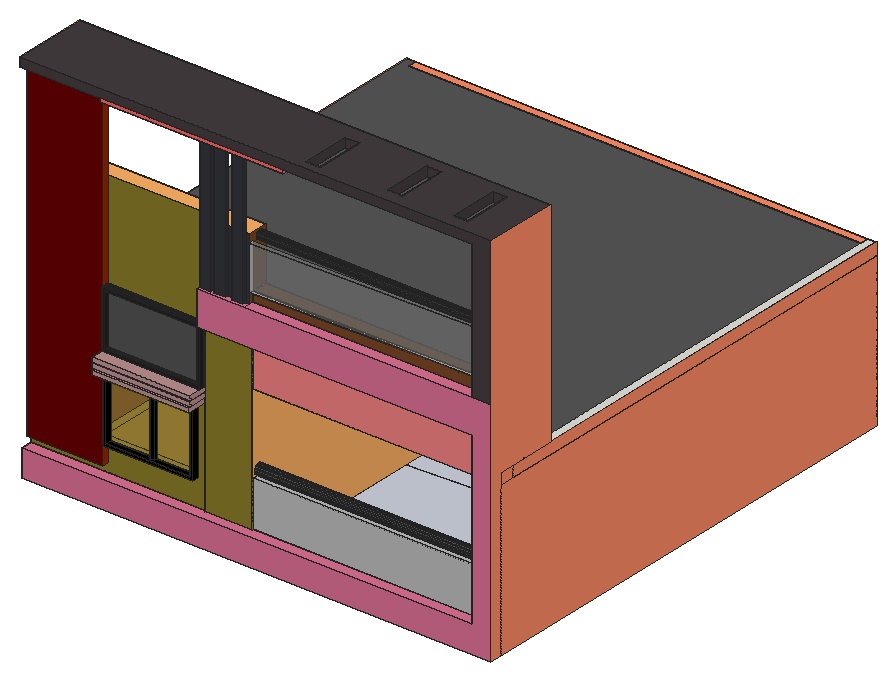
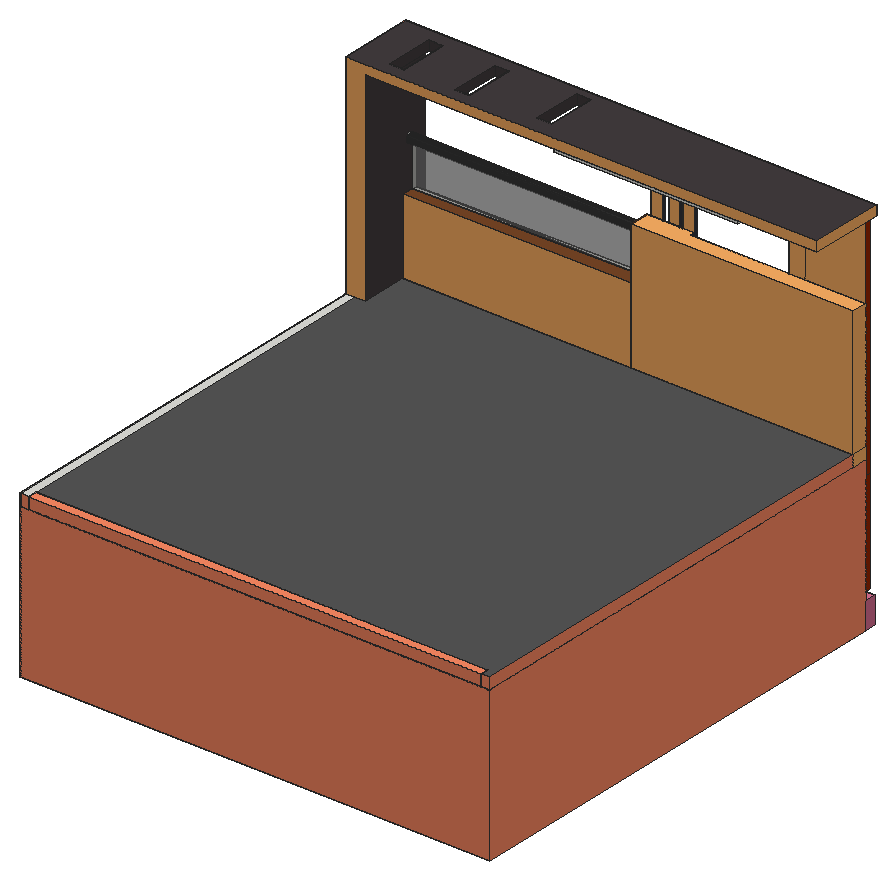
# SketchUp Ruby script. Lengths in inches.
U = 1.inch
M = Sketchup.active_model
def pt(a) = Geom::Point3d.new(a.map { |v| v * U })
def face(e, loops, mat)
  f = e.add_face(loops[0].map { |a| pt(a) })
  loops[1..].each { |l| e.add_face(l.map { |a| pt(a) }).erase! }
  f.material = f.back_material = mat if mat
  f
end
# faces: each face lists its corners as indices into pts; further lists are holes
def faces(e, pts, list, mat = nil) = list.each { |f| face(e, (f[0].is_a?(Array) ? f : [f]).map { |l| l.map { |i| pts[i] } }, mat) }
# xy, xz, yz: faces in a plane at the given z, y or x. An outline is a flat list of corners, or four numbers for a rectangle; further outlines are holes
def ring(l) = l.size == 4 ? [[l[0], l[1]], [l[2], l[1]], [l[2], l[3]], [l[0], l[3]]] : l.each_slice(2).to_a
def flat(e, list, mat, &to3) = list.each { |f| face(e, (f[0].is_a?(Array) ? f : [f]).map { |l| ring(l).map { |u, v| to3.(u, v) } }, mat) }
def xy(e, z, list, mat = nil) = flat(e, list, mat) { |x, y| [x, y, z] }
def xz(e, y, list, mat = nil) = flat(e, list, mat) { |x, z| [x, y, z] }
def yz(e, x, list, mat = nil) = flat(e, list, mat) { |y, z| [x, y, z] }
def lines(e, pts, list) = list.each { |a, b| e.add_line(pt(pts[a]), pt(pts[b])) }
# prism: a flat outline (further loops are holes) pulled along v
def prism(e, loops, v, mat = nil)
  f = face(e, loops, mat); d = Geom::Vector3d.new(v.map { |x| x * U })
  f.pushpull(f.normal.samedirection?(d) ? d.length : -d.length)
end
def box(e, o, s, mat = nil) = prism(e, [[o, [o[0] + s[0], o[1], o[2]], [o[0] + s[0], o[1] + s[1], o[2]], [o[0], o[1] + s[1], o[2]]]], [0, 0, s[2]], mat)
def at(x, y, z, deg = 0) = Geom::Transformation.translation(pt([x, y, z])) * Geom::Transformation.rotation(ORIGIN, Z_AXIS, deg.degrees)
def axes(o, x, y, z) = Geom::Transformation.new([*x, 0, *y, 0, *z, 0, *pt(o).to_a, 1])
def part(name) = M.definitions.add(name)
# library, detail: a bought-in or finely detailed component or shape, given as its bounding box
def library(name, o, s) = part(name).tap { |d| box(d.entities, o, s) }
def detail(e, o, s) = box(e.add_group.entities, o, s)
def put(e, d, t, mat = nil) = e.add_instance(d, t).tap { |i| i.material = mat if mat }
def group(e, t, mat = nil) = e.add_group.tap { |g| g.transformation = t; g.material = mat if mat }.entities
root = M.entities
M.materials.add("[0001_PaleVioletRed]").color = [219, 112, 147]
M.materials.add("[0013_LightCoral]").color = [240, 128, 128]
M.materials.add("[0119_RosyBrown]").color = [188, 143, 143]
M.materials.add("[0135_DarkGray]").color = [81, 81, 81]
M.materials.add("[0136_Charcoal]").color = [35, 35, 35]
M.materials.add("[Asphalt New]").color = [67, 60, 62]
M.materials.add("[Color A03]").color = [255, 101, 101]
M.materials.add("[Color A08]").color = [102, 0, 0]
M.materials.add("[Color B03]").color = [255, 140, 101]
M.materials.add("[Color B07]").color = [153, 38, 0]
M.materials.add("[Color C03]").color = [255, 178, 101]
M.materials.add("[Color M06]").color = [86, 86, 86]
M.materials.add("[Color M07]").color = [58, 58, 58]
M.materials.add("[Color M09]").color = [0, 0, 0]
M.materials.add("[Formica Laminate Dark]").color = [50, 53, 60]
M.materials.add("[Marble Carrara Floor Tile]").color = [204, 208, 219]
M.materials.add("[Mirror 01]").color = [185, 185, 185]
M.materials.add("[Translucent Glass Dark Green]").color = [62, 91, 5]
M.materials["[Translucent Glass Dark Green]"].alpha = 0.5
M.materials.add("[Translucent Glass Gray]").color = [128, 128, 128]
M.materials["[Translucent Glass Gray]"].alpha = 0.5
M.materials.add("[Wood Floor]").color = [155, 105, 61]
M.materials.add("[Wood Plywood Knots]").color = [137, 122, 41]
M.materials.add("[Wood Veneer 01]").color = [120, 70, 37]
c1 = library("glass+door",[0,-2.95,0],[39.37,5.9,82.68])
xy(root,156,[[472.5,7.75,481.5,19.75],[228.3125,215.25,228.3125,331.6875,272.65,331.6875,272.65,337.6875,222.3125,337.6875,222.3125,331.34],[430.11,331.6875,467.13,331.6875,466.82,337.6875,430.11,337.6875]])
xy(root,156,[[1.5,7.75,10.5,19.75],[10.5,7.75,10.5,19.75,179.9375,19.75,179.9375,18.75,228.3125,18.75,228.3125,19.75,472.5,19.75,472.5,7.75]],"[0001_PaleVioletRed]")
xy(root,156,[[[1.5,19.75,481.5,499.75],[10.5,28.75,472.5,28.75,472.5,331.6875,467.13,331.6875,466.82,337.6875,472.5,337.6875,472.5,490.75,10.5,490.75,10.5,221.25,222.3125,221.25,222.3125,331.34,228.3125,215.25,10.5,215.25]],[10.5,28.75,228.3125,215.25],[228.3125,28.75,228.3125,215.25,472.5,227.87,472.5,28.75]],"[Color C03]")
xy(root,156,[[228.3125,215.25,472.5,227.87,467.13,331.6875,430.11,331.6875,430.11,337.6875,472.5,337.6875,472.5,490.75,10.5,490.75,10.5,221.25,222.3125,221.25,222.3125,337.6875,272.65,337.6875,272.65,331.6875,228.3125,331.6875],[472.5,227.87,472.5,331.6875,467.13,331.6875]],"[Marble Carrara Floor Tile]")
xy(root,156.5,[[228.3125,28.75,472.5,28.75,472.5,227.87,228.3125,215.25]],"[Marble Carrara Floor Tile]")
xy(root,183.125,[[10.5,19.75,228.3125,28.75]])
xy(root,183.125,[[1.5,7.75,461.5625,19.75]],"[0001_PaleVioletRed]")
xy(root,191.625,[[1.5,13.75,63.75,19.75],[63.75,13.75,79.5,19.75]])
xy(root,210.02,[[79.5,13.75,171.875,19.75]])
xy(root,213.02,[[125.6875,16.75,129.85,19.75]])
xy(root,213.02,[[82.5,13.75,168.875,13.75,168.875,19.75,129.85,19.75,129.85,16.75,125.6875,16.75,125.6875,19.75,82.5,19.75]],"[Color M09]")
xy(root,230.125,[[228.3125,19.75,472.5,28.75]],"[Mirror 01]")
xy(root,253.3125,[[272.65,331.6875,430.11,337.6875]])
xy(root,271.2,[[125.6875,16.75,129.85,19.75]])
xy(root,271.2,[[82.5,13.75,82.5,19.75,125.6875,19.75,125.6875,16.75,129.85,16.75,129.85,19.75,168.875,19.75,168.875,13.75]],"[Color M09]")
xy(root,274.2,[[79.5,13.75,171.875,19.75]],"[Color M09]")
xy(root,281.13,[[79.5,0,178.52,19.75]],"[0119_RosyBrown]")
xy(root,285.75,[[79.5,0,178.45,19.75]],"[0119_RosyBrown]")
xy(root,286.88,[[79.5,0,180,19.75]],"[0119_RosyBrown]")
xy(root,291.5,[[79.5,0,179.9375,19.75]],"[0119_RosyBrown]")
xy(root,292.57,[[79.5,0,180,19.75]],"[0119_RosyBrown]")
xy(root,297.1875,[[79.5,12.4375,179.9375,15.4375],[79.5,15.4375,179.9375,19.75]])
xy(root,297.1875,[[79.5,0,179.9375,12.4375]],"[0119_RosyBrown]")
xy(root,300.53,[[82.84,12.4375,176.6,15.4375]],"[0136_Charcoal]")
xy(root,310.125,[[228.3125,35.87,472.5,331.6875]],"[0013_LightCoral]")
xy(root,311.9375,[[[1.5,35.87,1.5,499.75,481.5,499.75,481.5,35.87,472.5,35.87,472.5,331.6875,228.3125,331.6875,228.3125,35.87],[10.5,221.25,222.3125,221.25,222.3125,337.6875,472.5,337.6875,472.5,490.75,10.5,490.75]]])
xy(root,312,[[1.5,19.75,228.3125,35.87],[472.5,19.75,481.5,35.87],[1.5,35.87,228.3125,35.87,228.3125,221.25,10.5,221.25,10.5,490.75,10.375,490.75,10.375,499.75,1.5,499.75],[228.3125,35.87,472.5,221.25],[472.5,35.87,472.6875,221.25],
  [472.6875,35.87,481.25,499.75],[481.25,35.87,481.5,499.75],[10.5,221.25,10.5,490.75,472.5,490.75,472.5,337.6875,222.3125,337.6875,222.3125,221.25],[222.3125,221.25,228.3125,221.25,228.3125,331.6875,472.6875,331.6875,472.6875,337.6875,222.3125,337.6875],[228.3125,221.25,472.5,331.6875],
  [472.5,221.25,472.6875,331.6875],[472.5,337.6875,472.6875,490.75],[10.375,490.75,472.6875,499.75]])
xy(root,312,[[228.3125,19.75,472.5,35.87]],"[0013_LightCoral]")
xy(root,324,[[461.5625,19.75,481.5,35.87],[472.6875,35.87,481.25,83.5],[481.25,35.87,481.5,83.5],[472.6875,83.5,481.25,499.75],[481.25,83.5,481.5,499.75]])
xy(root,324,[[461.5625,35.87,472.6875,83.5],[10.375,490.75,472.6875,499.75]],"[Color B03]")
xy(root,324,[[1.5,35.87,461.5625,35.87,461.5625,83.5,472.6875,83.5,472.6875,490.75,10.375,490.75,10.375,499.75,1.5,499.75]],"[Color M06]")
xy(root,353.01,[[82.84,12.4375,176.6,15.4375]],"[0136_Charcoal]")
xy(root,356.35,[[179.9375,18.75,228.3125,19.75]])
xy(root,356.35,[[179.9375,7.75,179.9375,18.75,228.3125,18.75,228.3125,19.75,461.5625,19.75,461.5625,7.75]],"[0001_PaleVioletRed]")
xy(root,356.35,[[79.5,12.4375,179.9375,15.4375],[79.5,15.4375,179.9375,19.75]],"[0136_Charcoal]")
xy(root,391.1875,[[179.9375,12.0625,191.55,15.0625],[194.6875,12.0625,206.3,15],[212.625,12.0625,224.24,15],[179.9375,15.0625,228.3125,19.75]])
xy(root,391.1875,[[179.9375,7.75,228.3125,7.75,228.3125,15.0625,191.55,15.0625,191.55,12.0625,179.9375,12.0625],[228.3125,7.75,461.5625,19.75]],"[0001_PaleVioletRed]")
xy(root,401.375,[[228.41,15.3125,228.3125,19.75,440.6,19.75],[228.3125,19.75,440.6,19.75,460.84,20.17,460.75,24.61]])
xy(root,401.375,[[228.3125,19.75,460.75,24.61,460.84,20.17,440.6,19.75,461.5625,19.75,461.5625,35.87,228.3125,35.87]],"[Wood Veneer 01]")
xy(root,446.76,[[228.41,15.3125,460.84,20.17,460.75,24.61,228.3125,19.75]],"[Translucent Glass Gray]")
xy(root,455.5,[[179.9375,15.0625,228.3125,15.0625,228.3125,35.87,1.5,35.87,1.5,19.75,179.9375,19.75]],"[Color C03]")
xy(root,528.35,[[[80.95,7.75,268.72,83.5],[86.14,12.9375,263.53,78.3125]]],"[Color A03]")
xy(root,531.1875,[[1.5,13.75,79.5,19.75]])
xy(root,531.35,[[[80.95,7.75,268.72,83.5],[86.14,12.9375,263.53,78.3125],[179.9375,12.0625,191.55,15.0625]],[194.6875,12.0625,206.3,12.9375],[212.625,12.0625,224.24,12.9375],[179.9375,12.9375,191.55,15.0625],[194.6875,12.9375,206.3,15],
  [212.625,12.9375,224.24,15]])
xy(root,531.35,[[0,7.75,80.95,83.5],[[268.72,7.75,461.5625,83.5],[432.03,21.26,446.65,71.45],[365.09,21.26,379.71,71.45],[285.03,16.32,299.65,66.51]]],"[Asphalt New]")
xy(root,531.35,[[86.14,12.9375,86.14,78.3125,263.53,78.3125,263.53,12.9375,224.24,12.9375,224.24,15,212.625,15,212.625,12.9375,206.3,12.9375,206.3,15,194.6875,15,194.6875,12.9375,191.55,12.9375,191.55,15.0625,179.9375,15.0625,179.9375,12.9375]],"[Color A03]")
xy(root,541.0625,[[[0,7.75,481.5,83.5],[432.03,21.26,446.65,71.45],[365.09,21.26,379.71,71.45],[285.03,16.32,299.65,66.51]]],"[Asphalt New]")
xz(root,0,[[79.5,281.13,178.52,281.13,178.45,285.75,79.5,285.75],[79.5,286.88,180,286.88,179.9375,291.5,79.5,291.5],[79.5,292.57,180,292.57,179.9375,297.1875,79.5,297.1875]],"[0119_RosyBrown]")
xz(root,7.75,[[1.5,156,481.5,156,481.5,391.1875,179.9375,391.1875,179.9375,356.35,461.5625,356.35,461.5625,183.125,1.5,183.125]],"[0001_PaleVioletRed]")
xz(root,7.75,[[461.5625,391.1875,481.5,391.1875,481.5,541.0625,0,541.0625,0,531.35,461.5625,531.35]],"[Asphalt New]")
xz(root,7.75,[[80.95,528.35,268.72,531.35]],"[Color A03]")
xz(root,12.0625,[[179.9375,391.1875,191.55,531.35],[194.6875,391.1875,206.3,531.35],[212.625,391.1875,224.24,531.35]],"[Formica Laminate Dark]")
xz(root,12.4375,[[[79.5,297.1875,179.9375,356.35],[82.84,300.53,176.6,353.01]]],"[0136_Charcoal]")
xz(root,12.9375,[[86.14,528.35,263.53,531.35]],"[Color A03]")
xz(root,13.75,[[1.5,191.625,79.5,531.1875]],"[Color A08]")
xz(root,13.75,[[[79.5,210.02,171.875,274.2],[82.5,213.02,168.875,271.2]]],"[Color M09]")
xz(root,15,[[194.6875,391.1875,206.3,531.35],[212.625,391.1875,224.24,531.35]],"[Color C03]")
xz(root,15.0625,[[179.9375,455.5,191.55,531.35]],"[Color C03]")
xz(root,15.0625,[[191.55,391.1875,228.3125,455.5]],"[Formica Laminate Dark]")
xz(root,15.4375,[[[79.5,297.1875,179.9375,356.35],[82.84,300.53,176.6,353.01]]])
xz(root,15.4375,[[82.84,300.53,176.6,353.01]],"[0135_DarkGray]")
xz(root,16.32,[[285.03,531.35,299.65,541.0625]],"[Asphalt New]")
xz(root,16.75,[[125.6875,213.02,129.85,271.2]],"[Color M09]")
xz(root,18.75,[[179.9375,156,228.3125,356.35]],"[Wood Plywood Knots]")
xz(root,19.75,[[1.5,156,179.9375,183.125],[179.9375,156,228.3125,183.125],[228.3125,156,481.5,156,481.5,312,472.5,312,472.5,230.125,461.5625,230.125,461.5625,183.125,228.3125,183.125],[179.9375,183.125,179.9375,286.88,180,286.88,179.9375,291.5,179.9375,292.57,180,292.57,179.9375,297.1875,179.9375,312,228.3125,312,228.3125,183.125],[1.5,191.625,63.75,297.1875],
  [63.75,191.625,63.75,297.1875,79.5,297.1875,79.5,285.75,78.02,285.75,78.02,281.13,79.5,281.13,79.5,191.625],[[79.5,210.02,171.875,274.2],[82.5,213.02,168.875,271.2]],[125.6875,213.02,129.85,271.2],[461.5625,230.125,472.5,312],[78.02,281.13,79.5,285.75],
  [79.5,281.13,79.5,285.75,178.45,285.75,178.52,281.13],[79.5,286.88,179.9375,291.5],[179.9375,286.88,179.9375,291.5,180,286.88],[79.5,291.5,179.9375,292.57],[79.5,292.57,179.9375,297.1875],
  [179.9375,292.57,179.9375,297.1875,180,292.57],[1.5,297.1875,63.75,312],[63.75,297.1875,79.5,312],[79.5,297.1875,179.9375,312],[1.5,312,63.75,324],
  [63.75,312,79.5,324],[79.5,312,179.9375,324],[179.9375,312,228.3125,324],[461.5625,312,472.5,324],[472.5,312,481.5,324],
  [1.5,324,63.75,455.5],[63.75,324,79.5,455.5],[79.5,324,179.9375,356.35],[179.9375,324,228.3125,356.35],[179.9375,356.35,228.3125,391.1875],
  [228.3125,356.35,461.5625,391.1875]])
xz(root,19.75,[[228.3125,312,461.5625,356.35]],"[0013_LightCoral]")
xz(root,19.75,[[1.5,455.5,63.75,531.1875],[63.75,455.5,79.5,531.1875]],"[Color C03]")
xz(root,19.75,[[228.3125,183.125,461.5625,230.125]],"[Mirror 01]")
xz(root,19.75,[[82.5,213.02,125.6875,271.2],[129.85,213.02,168.875,271.2]],"[Translucent Glass Dark Green]")
xz(root,19.75,[[[1.5,183.125,179.9375,183.125,179.9375,286.88,79.5,286.88,79.5,297.1875,63.75,297.1875,63.75,191.625,1.5,191.625],[79.5,210.02,171.875,274.2],[78.02,281.13,78.02,285.75,178.45,285.75,178.52,281.13]],[79.5,356.35,179.9375,455.5]],"[Wood Plywood Knots]")
xz(root,19.75,[[228.3125,391.1875,461.5625,401.375]],"[Wood Veneer 01]")
xz(root,21.26,[[365.09,531.35,379.71,541.0625],[432.03,531.35,446.65,541.0625]],"[Asphalt New]")
xz(root,28.75,[[10.5,156,228.3125,183.125],[228.3125,156,472.5,156.5],[228.3125,156.5,472.5,230.125]])
xz(root,35.87,[[1.5,311.9375,228.3125,312],[472.5,311.9375,481.5,312],[1.5,312,228.3125,324],[228.3125,312,472.6875,324],[472.6875,312,481.25,324],
  [481.25,312,481.5,324]])
xz(root,35.87,[[228.3125,310.125,472.5,312]],"[0013_LightCoral]")
xz(root,35.87,[[1.5,324,228.3125,455.5],[228.3125,324,461.5625,401.375]],"[Color C03]")
xz(root,66.51,[[285.03,531.35,299.65,541.0625]],"[Asphalt New]")
xz(root,71.45,[[365.09,531.35,379.71,541.0625],[432.03,531.35,446.65,541.0625]],"[Asphalt New]")
xz(root,78.3125,[[86.14,528.35,263.53,531.35]],"[Color A03]")
xz(root,83.5,[[80.95,528.35,268.72,531.35]])
xz(root,83.5,[[461.5625,324,461.5625,531.35,0,531.35,0,541.0625,481.5,541.0625,481.5,324]],"[Color C03]")
xz(root,221.25,[[10.5,156,222.3125,311.9375],[10.5,311.9375,222.3125,312]])
xz(root,331.6875,[[228.3125,310.125,472.5,311.9375],[228.3125,311.9375,472.5,312]])
xz(root,331.6875,[[265.66,156,272.65,156,272.65,253.3125,430.11,253.3125,430.11,156,437.11,156,437.11,260.3125,265.66,260.3125]],"[Color B07]")
xz(root,331.6875,[[228.3125,156,265.66,156,265.66,260.3125,437.11,260.3125,437.11,156,472.5,156,472.5,310.125,228.3125,310.125]],"[Color C03]")
xz(root,337.6875,[[222.3125,156,222.3125,311.9375,472.5,311.9375,472.5,156,430.11,156,430.11,253.3125,272.65,253.3125,272.65,156],[222.3125,311.9375,472.5,312]])
xz(root,490.75,[[10.5,156,472.5,311.9375],[10.5,311.9375,472.5,312],[10.375,312,472.6875,324]])
xz(root,499.75,[[1.5,311.9375,481.5,312],[481.25,312,481.5,324]])
xz(root,499.75,[[1.5,156,481.5,311.9375],[1.5,312,10.375,324],[10.375,312,472.6875,324],[472.6875,312,481.25,324]],"[Color B03]")
yz(root,0,[[7.75,531.35,83.5,541.0625]],"[Color C03]")
yz(root,1.5,[[35.87,311.9375,499.75,312]])
yz(root,1.5,[[7.75,156,19.75,183.125]],"[0001_PaleVioletRed]")
yz(root,1.5,[[19.75,156,19.75,312,35.87,312,35.87,311.9375,499.75,311.9375,499.75,156],[35.87,312,499.75,324]],"[Color B03]")
yz(root,1.5,[[13.75,191.625,19.75,297.1875],[13.75,297.1875,19.75,531.1875]],"[Color B07]")
yz(root,1.5,[[19.75,312,35.87,324],[19.75,324,35.87,455.5]],"[Color C03]")
yz(root,10.375,[[490.75,312,499.75,324]])
yz(root,10.5,[[221.25,156,490.75,311.9375],[221.25,311.9375,490.75,312]])
yz(root,79.5,[[13.75,210.02,19.75,274.2],[13.75,274.2,19.75,281.13],[13.75,281.13,19.75,285.75],[13.75,285.75,19.75,286.88],[13.75,286.88,19.75,291.5],
  [13.75,291.5,19.75,292.57],[13.75,292.57,19.75,297.1875],[13.75,297.1875,15.4375,356.35],[15.4375,297.1875,19.75,356.35]])
yz(root,79.5,[[0,281.13,13.75,285.75],[0,286.88,13.75,291.5],[0,292.57,13.75,297.1875]],"[0119_RosyBrown]")
yz(root,79.5,[[12.4375,297.1875,13.75,356.35]],"[0136_Charcoal]")
yz(root,79.5,[[13.75,191.625,19.75,210.02],[13.75,356.35,19.75,531.1875]],"[Color B07]")
yz(root,80.95,[[7.75,528.35,83.5,531.35]])
yz(root,82.5,[[13.75,213.02,19.75,271.2]],"[Color M09]")
yz(root,82.84,[[12.4375,300.53,15.4375,353.01]],"[0136_Charcoal]")
yz(root,86.14,[[12.9375,528.35,78.3125,531.35]],"[Color A03]")
yz(root,125.6875,[[16.75,213.02,19.75,271.2]],"[Color M09]")
yz(root,129.85,[[16.75,213.02,19.75,271.2]],"[Color M09]")
yz(root,168.875,[[13.75,213.02,19.75,271.2]],"[Color M09]")
yz(root,171.875,[[13.75,210.02,19.75,274.2]],"[Color M09]")
yz(root,176.6,[[12.4375,300.53,15.4375,353.01]],"[0136_Charcoal]")
yz(root,179.9375,[[18.75,156,19.75,291.5],[18.75,291.5,19.75,297.1875],[18.75,297.1875,19.75,324],[18.75,324,19.75,356.35]])
yz(root,179.9375,[[7.75,356.35,19.75,391.1875]],"[0001_PaleVioletRed]")
yz(root,179.9375,[[12.4375,297.1875,15.4375,356.35],[15.4375,297.1875,18.75,356.35]],"[0136_Charcoal]")
yz(root,179.9375,[[12.0625,391.1875,12.0625,531.35,15.0625,531.35,15.0625,455.5,19.75,455.5,19.75,391.1875]],"[Formica Laminate Dark]")
yz(root,191.55,[[12.0625,391.1875,15.0625,531.35]],"[Formica Laminate Dark]")
yz(root,194.6875,[[12.0625,391.1875,15,531.35]],"[Formica Laminate Dark]")
yz(root,206.3,[[12.0625,391.1875,15,531.35]],"[Formica Laminate Dark]")
yz(root,212.625,[[12.0625,391.1875,15,531.35]],"[Formica Laminate Dark]")
yz(root,222.3125,[[221.25,156,337.6875,311.9375],[221.25,311.9375,337.6875,312]])
yz(root,224.24,[[12.0625,391.1875,15,531.35]],"[Formica Laminate Dark]")
yz(root,228.3125,[[28.75,156,215.25,156.5],[19.75,183.125,28.75,230.125],[35.87,310.125,331.6875,311.9375],[35.87,311.9375,331.6875,312],[19.75,312,35.87,401.375]])
yz(root,228.3125,[[[215.25,156,331.6875,156,331.6875,310.125,35.87,310.125,35.87,312,19.75,312,19.75,230.125,28.75,230.125,28.75,156.5,215.25,156.5],[26.28,230.8,24.95,230.97,23.71,231.48,22.65,232.3,21.84,233.36,21.33,234.6,21.15,235.92,21.33,237.25,21.84,238.49,22.65,239.55,23.71,240.36,24.95,240.87,26.28,241.05,27.6,240.87,28.84,240.36,29.9,239.55,30.72,238.49,31.23,237.25,31.4,235.92,31.23,234.6,30.72,233.36,29.9,232.3,28.84,231.48,27.6,230.97]]],"[Color C03]")
yz(root,228.3125,[[18.75,156,19.75,356.35]],"[Wood Plywood Knots]")
yz(root,228.3125,[[[15.0625,391.1875,19.75,391.1875,19.75,401.375,35.87,401.375,35.87,455.5,15.0625,455.5],[27.79,445.44,26.63,445.59,25.54,446.04,24.61,446.76,23.89,447.69,23.45,448.77,23.29,449.94,23.45,451.1,23.89,452.19,24.61,453.12,25.54,453.84,26.63,454.29,27.79,454.44,28.96,454.29,30.04,453.84,30.97,453.12,31.6875,452.19,32.14,451.1,32.29,449.94,32.14,448.77,31.6875,447.69,30.97,446.76,30.04,446.04,28.96,445.59]]],"[Wood Veneer 01]")
yz(root,263.53,[[12.9375,528.35,78.3125,531.35]],"[Color A03]")
yz(root,268.72,[[7.75,528.35,83.5,531.35]],"[Color A03]")
yz(root,272.65,[[331.6875,156,337.6875,253.3125]],"[Color B07]")
yz(root,285.03,[[16.32,531.35,66.51,541.0625]],"[Asphalt New]")
yz(root,299.65,[[16.32,531.35,66.51,541.0625]],"[Asphalt New]")
yz(root,365.09,[[21.26,531.35,71.45,541.0625]],"[Asphalt New]")
yz(root,379.71,[[21.26,531.35,71.45,541.0625]],"[Asphalt New]")
yz(root,430.11,[[331.6875,156,337.6875,253.3125]],"[Color B07]")
yz(root,432.03,[[21.26,531.35,71.45,541.0625]],"[Asphalt New]")
yz(root,446.65,[[21.26,531.35,71.45,541.0625]],"[Asphalt New]")
yz(root,460.75,[[27.79,445.44,28.96,445.59,30.04,446.04,30.97,446.76,31.6875,447.69,32.14,448.77,32.29,449.94,32.14,451.1,31.6875,452.19,30.97,453.12,30.04,453.84,28.96,454.29,27.79,454.44,26.63,454.29,25.54,453.84,24.61,453.12,23.89,452.19,23.45,451.1,23.29,449.94,23.45,448.77,23.89,447.69,24.61,446.76,25.54,446.04,26.63,445.59]])
yz(root,461.5625,[[26.28,230.8,27.6,230.97,28.84,231.48,29.9,232.3,30.72,233.36,31.23,234.6,31.4,235.92,31.23,237.25,30.72,238.49,29.9,239.55,28.84,240.36,27.6,240.87,26.28,241.05,24.95,240.87,23.71,240.36,22.65,239.55,21.84,238.49,21.33,237.25,21.15,235.92,21.33,234.6,21.84,233.36,22.65,232.3,23.71,231.48,24.95,230.97],[19.75,324,35.87,401.375]])
yz(root,461.5625,[[7.75,183.125,19.75,356.35]],"[0001_PaleVioletRed]")
yz(root,461.5625,[[35.87,324,35.87,401.375,19.75,401.375,19.75,391.1875,7.75,391.1875,7.75,531.35,83.5,531.35,83.5,324]],"[Asphalt New]")
yz(root,472.5,[[28.75,156,227.87,156.5],[337.6875,156,490.75,311.9375],[19.75,230.125,28.75,312],[35.87,310.125,331.6875,311.9375],[35.87,311.9375,331.6875,312],
  [337.6875,311.9375,490.75,312]])
yz(root,472.5,[[227.87,156,227.87,156.5,28.75,156.5,28.75,312,35.87,312,35.87,310.125,331.6875,310.125,331.6875,156]],"[Color C03]")
yz(root,472.6875,[[490.75,312,499.75,324]])
yz(root,481.25,[[35.87,312,499.75,324]])
yz(root,481.5,[[35.87,311.9375,499.75,312]])
yz(root,481.5,[[7.75,156,19.75,156,19.75,324,83.5,324,83.5,541.0625,7.75,541.0625],[19.75,156,499.75,156,499.75,311.9375,35.87,311.9375,35.87,312,19.75,312],[19.75,312,35.87,324],[35.87,312,499.75,324]],"[Color B03]")
p = [[262.87,217.04,148.37],[262.87,217.04,145.06],[457.11,227.08,145.06],[457.11,227.08,148.37],[472.5,227.87,156],[228.3125,215.25,156],
  [228.3125,215.25,156.5],[472.5,227.87,156.5],[228.3125,24.95,230.97],[228.3125,26.28,230.8],[461.5625,26.28,230.8],[461.5625,24.95,230.97],
  [228.3125,27.6,230.97],[461.5625,27.6,230.97],[228.3125,23.71,231.48],[461.5625,23.71,231.48],[228.3125,28.84,231.48],[461.5625,28.84,231.48],
  [228.3125,22.65,232.3],[461.5625,22.65,232.3],[228.3125,29.9,232.3],[461.5625,29.9,232.3],[228.3125,21.84,233.36],[461.5625,21.84,233.36],
  [228.3125,30.72,233.36],[461.5625,30.72,233.36],[228.3125,21.33,234.6],[461.5625,21.33,234.6],[228.3125,31.23,234.6],[461.5625,31.23,234.6],
  [228.3125,21.15,235.92],[461.5625,21.15,235.92],[228.3125,31.4,235.92],[461.5625,31.4,235.92],[228.3125,21.33,237.25],[461.5625,21.33,237.25],
  [228.3125,31.23,237.25],[461.5625,31.23,237.25],[228.3125,21.84,238.49],[461.5625,21.84,238.49],[228.3125,30.72,238.49],[461.5625,30.72,238.49],
  [228.3125,22.65,239.55],[461.5625,22.65,239.55],[228.3125,29.9,239.55],[461.5625,29.9,239.55],[228.3125,23.71,240.36],[461.5625,23.71,240.36],
  [228.3125,28.84,240.36],[461.5625,28.84,240.36],[228.3125,24.95,240.87],[461.5625,24.95,240.87],[228.3125,27.6,240.87],[461.5625,27.6,240.87],
  [228.3125,26.28,241.05],[461.5625,26.28,241.05],[178.52,19.75,281.13],[178.45,19.75,285.75],[178.45,0,285.75],[178.52,0,281.13],
  [180,19.75,286.88],[179.9375,19.75,291.5],[179.9375,18.75,291.5],[179.9375,0,291.5],[180,0,286.88],[180,19.75,292.57],
  [179.9375,19.75,297.1875],[179.9375,18.75,297.1875],[179.9375,15.4375,297.1875],[179.9375,12.4375,297.1875],[179.9375,0,297.1875],[180,0,292.57],
  [228.3125,19.75,446.76],[228.3125,19.75,401.375],[228.41,15.3125,401.375],[228.41,15.3125,446.76],[440.6,19.75,401.375],[460.84,20.17,401.375],
  [460.84,20.17,446.76],[460.75,24.61,401.375],[460.75,24.61,446.76],[228.3125,26.63,445.59],[228.3125,27.79,445.44],[460.75,27.79,445.44],
  [460.75,26.63,445.59],[228.3125,28.96,445.59],[460.75,28.96,445.59],[228.3125,25.54,446.04],[460.75,25.54,446.04],[228.3125,30.04,446.04],
  [460.75,30.04,446.04],[228.3125,24.61,446.76],[228.3125,30.97,446.76],[460.75,30.97,446.76],[228.3125,23.89,447.69],[460.75,23.89,447.69],
  [228.3125,31.6875,447.69],[460.75,31.6875,447.69],[228.3125,23.45,448.77],[460.75,23.45,448.77],[228.3125,32.14,448.77],[460.75,32.14,448.77],
  [228.3125,23.29,449.94],[460.75,23.29,449.94],[228.3125,32.29,449.94],[460.75,32.29,449.94],[228.3125,23.45,451.1],[460.75,23.45,451.1],
  [228.3125,32.14,451.1],[460.75,32.14,451.1],[228.3125,23.89,452.19],[460.75,23.89,452.19],[228.3125,31.6875,452.19],[460.75,31.6875,452.19],
  [228.3125,24.61,453.12],[460.75,24.61,453.12],[228.3125,30.97,453.12],[460.75,30.97,453.12],[228.3125,25.54,453.84],[460.75,25.54,453.84],
  [228.3125,30.04,453.84],[460.75,30.04,453.84],[228.3125,26.63,454.29],[460.75,26.63,454.29],[228.3125,28.96,454.29],[460.75,28.96,454.29],
  [228.3125,27.79,454.44],[460.75,27.79,454.44],[228.3125,33.875,202.625],[10.5,33.875,202.625],[10.5,40.375,202.625],[228.3125,40.375,202.625],
  [10.5,40.375,183.125],[228.3125,40.375,183.125],[10.5,19.75,202.625],[10.5,28.75,183.125],[10.5,33.875,312]]
faces(root,p,[[0,1,2,3]],"[Wood Floor]")
faces(root,p,[[4,5,6,7],[72,73,74,75],[79,80,78,77]])
faces(root,p,[[8,9,10,11],[9,12,13,10],[14,8,11,15],[12,16,17,13],[18,14,15,19],[16,20,21,17],[22,18,19,23],[20,24,25,21],
  [26,22,23,27],[24,28,29,25],[30,26,27,31],[28,32,33,29],[34,30,31,35],[32,36,37,33],[38,34,35,39],[36,40,41,37],
  [42,38,39,43],[40,44,45,41],[46,42,43,47],[44,48,49,45],[50,46,47,51],[48,52,53,49],[54,50,51,55],[52,54,55,53]],"[Color M06]")
faces(root,p,[[56,57,58,59],[60,61,62,63,64],[65,66,67,68,69,70,71]],"[0119_RosyBrown]")
faces(root,p,[[74,76,77,78,75],[79,73,72,80]],"[Translucent Glass Gray]")
faces(root,p,[[81,82,83,84],[82,85,86,83],[87,81,84,88],[85,89,90,86],[91,87,88,80],[89,92,93,90],[94,91,80,95],[92,96,97,93],
  [98,94,95,99],[96,100,101,97],[102,98,99,103],[100,104,105,101],[106,102,103,107],[104,108,109,105],[110,106,107,111],[108,112,113,109],
  [114,110,111,115],[112,116,117,113],[118,114,115,119],[116,120,121,117],[122,118,119,123],[120,124,125,121],[126,122,123,127],[124,126,127,125]],"[Color M07]")
lines(root,p,[[128,129],[130,131],[132,133],[132,130],[134,129],[135,132],[129,130],[129,136]])
put(root,c1,axes([272.65,331.1875,156],[3.97579,0,0],[0,1.17,0],[0,0,1.17]))
